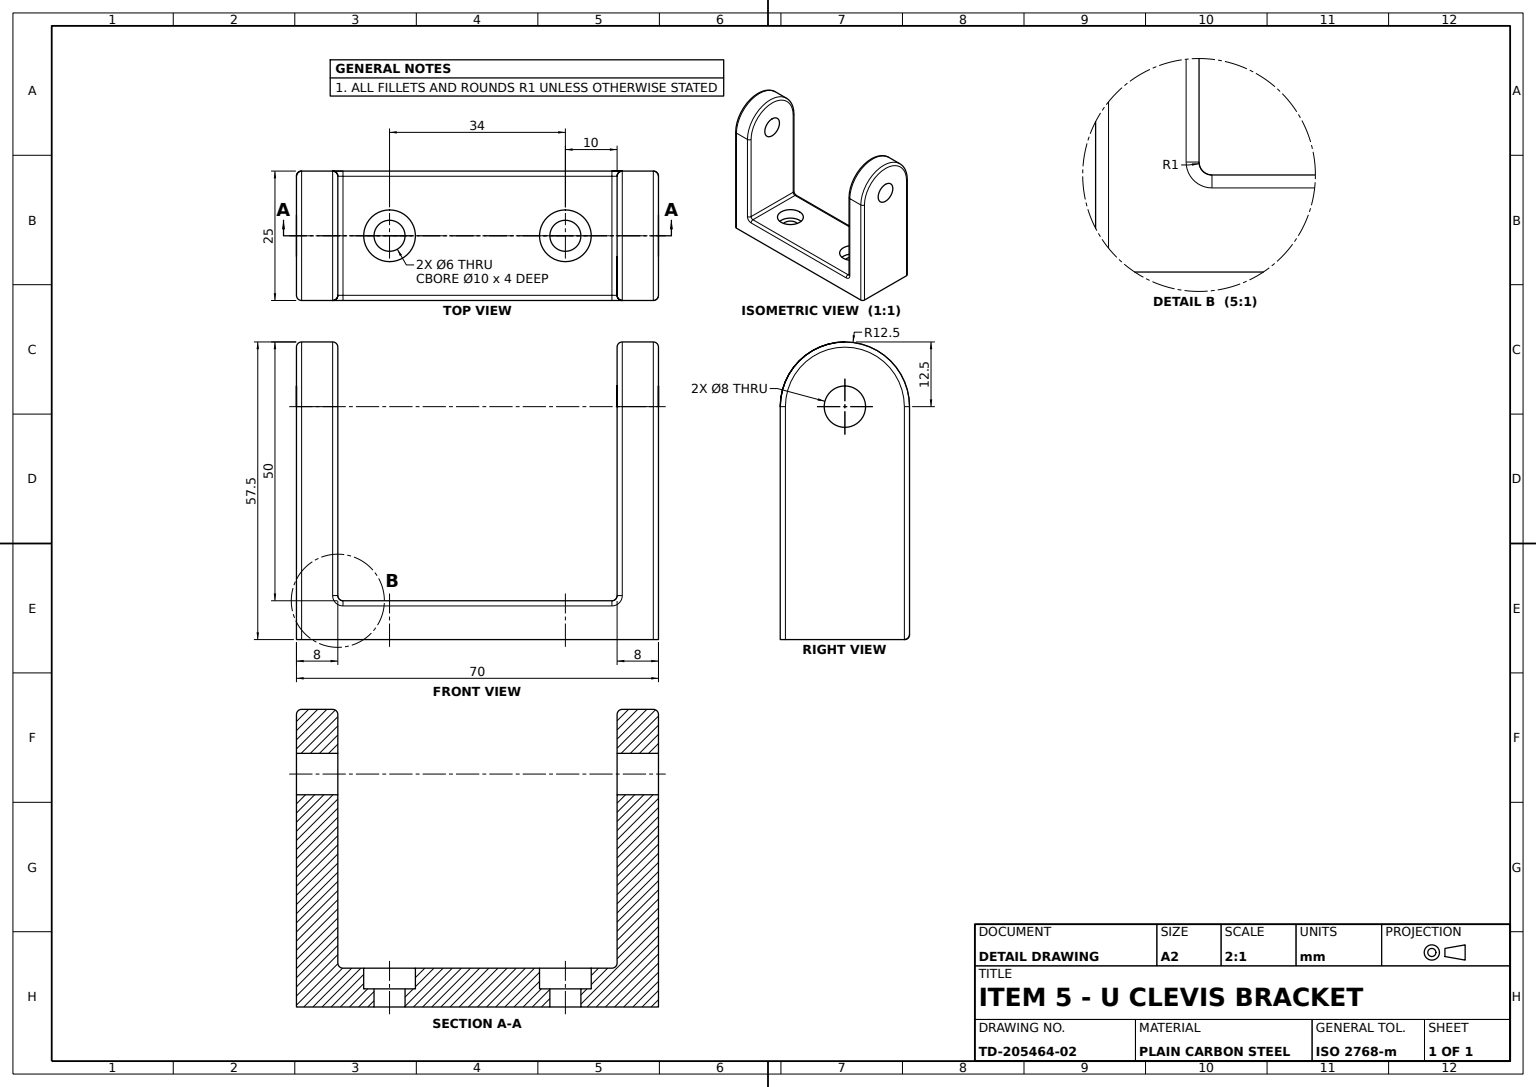
ISO-10303-21;
HEADER;
FILE_DESCRIPTION((''),'2;1');
FILE_NAME('','',(''),(''),'','','');
FILE_SCHEMA(('AUTOMOTIVE_DESIGN'));
ENDSEC;
DATA;
#1=APPLICATION_CONTEXT('');
#2=PRODUCT_CONTEXT('',#1,'mechanical');
#3=PRODUCT('','','',(#2));
#4=PRODUCT_DEFINITION_FORMATION('','',#3);
#5=PRODUCT_DEFINITION_CONTEXT('',#1,'design');
#6=PRODUCT_DEFINITION('','',#4,#5);
#7=PRODUCT_DEFINITION_SHAPE('','',#6);
#8=(LENGTH_UNIT()NAMED_UNIT(*)SI_UNIT(.MILLI.,.METRE.));
#9=(NAMED_UNIT(*)PLANE_ANGLE_UNIT()SI_UNIT($,.RADIAN.));
#10=(NAMED_UNIT(*)SI_UNIT($,.STERADIAN.)SOLID_ANGLE_UNIT());
#11=UNCERTAINTY_MEASURE_WITH_UNIT(LENGTH_MEASURE(1.E-05),#8,'distance_accuracy_value','');
#12=(GEOMETRIC_REPRESENTATION_CONTEXT(3)GLOBAL_UNCERTAINTY_ASSIGNED_CONTEXT((#11))GLOBAL_UNIT_ASSIGNED_CONTEXT((#8,#9,#10))REPRESENTATION_CONTEXT('',''));
#13=CARTESIAN_POINT('',(35.,41.,0.));
#14=VERTEX_POINT('',#13);
#15=CARTESIAN_POINT('',(35.,49.,0.));
#16=VERTEX_POINT('',#15);
#17=CARTESIAN_POINT('',(35.,45.,0.));
#18=DIRECTION('',(-1.,0.,0.));
#19=DIRECTION('',(0.,-1.,0.));
#20=AXIS2_PLACEMENT_3D('',#17,#18,#19);
#21=CIRCLE('',#20,4.);
#22=EDGE_CURVE('',#14,#16,#21,.T.);
#23=ORIENTED_EDGE('',*,*,#22,.F.);
#24=CARTESIAN_POINT('',(27.,41.,0.));
#25=VERTEX_POINT('',#24);
#26=VECTOR('',#18,1000.);
#27=LINE('',#13,#26);
#28=EDGE_CURVE('',#14,#25,#27,.T.);
#29=ORIENTED_EDGE('',*,*,#28,.T.);
#30=CARTESIAN_POINT('',(27.,49.,0.));
#31=VERTEX_POINT('',#30);
#32=CARTESIAN_POINT('',(27.,45.,0.));
#33=DIRECTION('',(1.,0.,0.));
#34=DIRECTION('',(0.,1.,0.));
#35=AXIS2_PLACEMENT_3D('',#32,#33,#34);
#36=CIRCLE('',#35,4.);
#37=EDGE_CURVE('',#31,#25,#36,.T.);
#38=ORIENTED_EDGE('',*,*,#37,.F.);
#39=LINE('',#15,#26);
#40=EDGE_CURVE('',#16,#31,#39,.T.);
#41=ORIENTED_EDGE('',*,*,#40,.F.);
#42=EDGE_LOOP('',(#23,#29,#38,#41));
#43=FACE_OUTER_BOUND('',#42,.T.);
#44=CYLINDRICAL_SURFACE('',#20,4.);
#45=ADVANCED_FACE('',(#43),#44,.F.);
#46=CARTESIAN_POINT('',(-27.,49.,0.));
#47=VERTEX_POINT('',#46);
#48=CARTESIAN_POINT('',(-35.,49.,0.));
#49=VERTEX_POINT('',#48);
#50=EDGE_CURVE('',#47,#49,#39,.T.);
#51=ORIENTED_EDGE('',*,*,#50,.F.);
#52=CARTESIAN_POINT('',(-27.,41.,0.));
#53=VERTEX_POINT('',#52);
#54=CARTESIAN_POINT('',(-27.,45.,0.));
#55=AXIS2_PLACEMENT_3D('',#54,#18,#19);
#56=CIRCLE('',#55,4.);
#57=EDGE_CURVE('',#53,#47,#56,.T.);
#58=ORIENTED_EDGE('',*,*,#57,.F.);
#59=CARTESIAN_POINT('',(-35.,41.,0.));
#60=VERTEX_POINT('',#59);
#61=EDGE_CURVE('',#53,#60,#27,.T.);
#62=ORIENTED_EDGE('',*,*,#61,.T.);
#63=CARTESIAN_POINT('',(-35.,45.,0.));
#64=AXIS2_PLACEMENT_3D('',#63,#18,#19);
#65=CIRCLE('',#64,4.);
#66=EDGE_CURVE('',#60,#49,#65,.T.);
#67=ORIENTED_EDGE('',*,*,#66,.T.);
#68=EDGE_LOOP('',(#51,#58,#62,#67));
#69=FACE_OUTER_BOUND('',#68,.T.);
#70=ADVANCED_FACE('',(#69),#44,.F.);
#71=CARTESIAN_POINT('',(-35.,0.,-11.5));
#72=VERTEX_POINT('',#71);
#73=CARTESIAN_POINT('',(35.,0.,-11.5));
#74=VERTEX_POINT('',#73);
#75=VECTOR('',#33,1000.);
#76=LINE('',#73,#75);
#77=EDGE_CURVE('',#72,#74,#76,.T.);
#78=ORIENTED_EDGE('',*,*,#77,.F.);
#79=CARTESIAN_POINT('',(-34.,1.,-12.5));
#80=VERTEX_POINT('',#79);
#81=CARTESIAN_POINT('',(-34.585786,0.414214,-12.5));
#82=CARTESIAN_POINT('',(-35.,0.,-12.085786));
#83=(BOUNDED_CURVE()B_SPLINE_CURVE(3,(#79,#81,#82,#71),.UNSPECIFIED.,.F.,.T.)B_SPLINE_CURVE_WITH_KNOTS((4,4),(1.570796327,3.141592654),.UNSPECIFIED.)CURVE()GEOMETRIC_REPRESENTATION_ITEM()RATIONAL_B_SPLINE_CURVE((1.,0.804737854,0.804737854,1.))REPRESENTATION_ITEM(''));
#84=EDGE_CURVE('',#80,#72,#83,.T.);
#85=ORIENTED_EDGE('',*,*,#84,.F.);
#86=CARTESIAN_POINT('',(34.,1.,-12.5));
#87=VERTEX_POINT('',#86);
#88=CARTESIAN_POINT('',(0.,1.,-12.5));
#89=LINE('',#88,#26);
#90=EDGE_CURVE('',#87,#80,#89,.T.);
#91=ORIENTED_EDGE('',*,*,#90,.F.);
#92=CARTESIAN_POINT('',(34.585786,0.414214,-12.5));
#93=CARTESIAN_POINT('',(35.,0.,-12.085786));
#94=(BOUNDED_CURVE()B_SPLINE_CURVE(3,(#86,#92,#93,#73),.UNSPECIFIED.,.F.,.F.)B_SPLINE_CURVE_WITH_KNOTS((4,4),(1.570796327,3.141592654),.UNSPECIFIED.)CURVE()GEOMETRIC_REPRESENTATION_ITEM()RATIONAL_B_SPLINE_CURVE((1.,0.804737854,0.804737854,1.))REPRESENTATION_ITEM(''));
#95=EDGE_CURVE('',#87,#74,#94,.T.);
#96=ORIENTED_EDGE('',*,*,#95,.T.);
#97=EDGE_LOOP('',(#78,#85,#91,#96));
#98=FACE_OUTER_BOUND('',#97,.T.);
#99=CARTESIAN_POINT('',(35.,1.,-11.5));
#100=AXIS2_PLACEMENT_3D('',#99,#33,#34);
#101=CYLINDRICAL_SURFACE('',#100,1.);
#102=ADVANCED_FACE('',(#98),#101,.T.);
#103=CARTESIAN_POINT('',(28.,8.5,-12.5));
#104=VERTEX_POINT('',#103);
#105=CARTESIAN_POINT('',(26.,6.5,-12.5));
#106=VERTEX_POINT('',#105);
#107=CARTESIAN_POINT('',(26.,8.5,-12.5));
#108=DIRECTION('',(0.,0.,-1.));
#109=AXIS2_PLACEMENT_3D('',#107,#108,#33);
#110=CIRCLE('',#109,2.);
#111=EDGE_CURVE('',#104,#106,#110,.T.);
#112=ORIENTED_EDGE('',*,*,#111,.F.);
#113=CARTESIAN_POINT('',(28.,45.,-12.5));
#114=VERTEX_POINT('',#113);
#115=CARTESIAN_POINT('',(28.,0.,-12.5));
#116=VECTOR('',#34,1000.);
#117=LINE('',#115,#116);
#118=EDGE_CURVE('',#104,#114,#117,.T.);
#119=ORIENTED_EDGE('',*,*,#118,.T.);
#120=CARTESIAN_POINT('',(34.,45.,-12.5));
#121=VERTEX_POINT('',#120);
#122=CARTESIAN_POINT('',(0.,45.,-12.5));
#123=LINE('',#122,#75);
#124=EDGE_CURVE('',#114,#121,#123,.T.);
#125=ORIENTED_EDGE('',*,*,#124,.T.);
#126=CARTESIAN_POINT('',(34.,0.,-12.5));
#127=VECTOR('',#19,1000.);
#128=LINE('',#126,#127);
#129=EDGE_CURVE('',#121,#87,#128,.T.);
#130=ORIENTED_EDGE('',*,*,#129,.T.);
#131=ORIENTED_EDGE('',*,*,#90,.T.);
#132=CARTESIAN_POINT('',(-34.,45.,-12.5));
#133=VERTEX_POINT('',#132);
#134=CARTESIAN_POINT('',(-34.,0.,-12.5));
#135=LINE('',#134,#116);
#136=EDGE_CURVE('',#80,#133,#135,.T.);
#137=ORIENTED_EDGE('',*,*,#136,.T.);
#138=CARTESIAN_POINT('',(-28.,45.,-12.5));
#139=VERTEX_POINT('',#138);
#140=EDGE_CURVE('',#133,#139,#123,.T.);
#141=ORIENTED_EDGE('',*,*,#140,.T.);
#142=CARTESIAN_POINT('',(-28.,8.5,-12.5));
#143=VERTEX_POINT('',#142);
#144=CARTESIAN_POINT('',(-28.,0.,-12.5));
#145=LINE('',#144,#127);
#146=EDGE_CURVE('',#139,#143,#145,.T.);
#147=ORIENTED_EDGE('',*,*,#146,.T.);
#148=CARTESIAN_POINT('',(-26.,6.5,-12.5));
#149=VERTEX_POINT('',#148);
#150=CARTESIAN_POINT('',(-26.,8.5,-12.5));
#151=AXIS2_PLACEMENT_3D('',#150,#108,#33);
#152=CIRCLE('',#151,2.);
#153=EDGE_CURVE('',#149,#143,#152,.T.);
#154=ORIENTED_EDGE('',*,*,#153,.F.);
#155=CARTESIAN_POINT('',(0.,6.5,-12.5));
#156=LINE('',#155,#75);
#157=EDGE_CURVE('',#149,#106,#156,.T.);
#158=ORIENTED_EDGE('',*,*,#157,.T.);
#159=EDGE_LOOP('',(#112,#119,#125,#130,#131,#137,#141,#147,#154,#158));
#160=FACE_OUTER_BOUND('',#159,.T.);
#161=CARTESIAN_POINT('',(0.,0.,-12.5));
#162=DIRECTION('',(0.,0.,1.));
#163=AXIS2_PLACEMENT_3D('',#161,#162,#33);
#164=PLANE('',#163);
#165=ADVANCED_FACE('',(#160),#164,.F.);
#166=CARTESIAN_POINT('',(17.,0.,3.));
#167=VERTEX_POINT('',#166);
#168=CARTESIAN_POINT('',(17.,3.5,3.));
#169=VERTEX_POINT('',#168);
#170=LINE('',#166,#116);
#171=EDGE_CURVE('',#167,#169,#170,.T.);
#172=ORIENTED_EDGE('',*,*,#171,.F.);
#173=CARTESIAN_POINT('',(17.,0.,-3.));
#174=VERTEX_POINT('',#173);
#175=CARTESIAN_POINT('',(17.,0.,0.));
#176=AXIS2_PLACEMENT_3D('',#175,#34,#162);
#177=CIRCLE('',#176,3.);
#178=EDGE_CURVE('',#174,#167,#177,.T.);
#179=ORIENTED_EDGE('',*,*,#178,.F.);
#180=CARTESIAN_POINT('',(17.,3.5,-3.));
#181=VERTEX_POINT('',#180);
#182=LINE('',#173,#116);
#183=EDGE_CURVE('',#174,#181,#182,.T.);
#184=ORIENTED_EDGE('',*,*,#183,.T.);
#185=CARTESIAN_POINT('',(17.,3.5,0.));
#186=AXIS2_PLACEMENT_3D('',#185,#34,#162);
#187=CIRCLE('',#186,3.);
#188=EDGE_CURVE('',#181,#169,#187,.T.);
#189=ORIENTED_EDGE('',*,*,#188,.T.);
#190=EDGE_LOOP('',(#172,#179,#184,#189));
#191=FACE_OUTER_BOUND('',#190,.T.);
#192=CYLINDRICAL_SURFACE('',#176,3.);
#193=ADVANCED_FACE('',(#191),#192,.F.);
#194=CARTESIAN_POINT('',(-34.,0.,12.5));
#195=VERTEX_POINT('',#194);
#196=CARTESIAN_POINT('',(-35.,0.,11.5));
#197=VERTEX_POINT('',#196);
#198=CARTESIAN_POINT('',(-34.,0.,11.5));
#199=AXIS2_PLACEMENT_3D('',#198,#19,#18);
#200=CIRCLE('',#199,1.);
#201=EDGE_CURVE('',#195,#197,#200,.T.);
#202=ORIENTED_EDGE('',*,*,#201,.F.);
#203=CARTESIAN_POINT('',(-34.,45.,12.5));
#204=VERTEX_POINT('',#203);
#205=LINE('',#194,#127);
#206=EDGE_CURVE('',#204,#195,#205,.T.);
#207=ORIENTED_EDGE('',*,*,#206,.F.);
#208=CARTESIAN_POINT('',(-35.,45.,11.5));
#209=VERTEX_POINT('',#208);
#210=CARTESIAN_POINT('',(-34.,45.,11.5));
#211=AXIS2_PLACEMENT_3D('',#210,#19,#108);
#212=CIRCLE('',#211,1.);
#213=EDGE_CURVE('',#204,#209,#212,.T.);
#214=ORIENTED_EDGE('',*,*,#213,.T.);
#215=LINE('',#208,#116);
#216=EDGE_CURVE('',#197,#209,#215,.T.);
#217=ORIENTED_EDGE('',*,*,#216,.F.);
#218=EDGE_LOOP('',(#202,#207,#214,#217));
#219=FACE_OUTER_BOUND('',#218,.T.);
#220=AXIS2_PLACEMENT_3D('',#198,#34,#162);
#221=CYLINDRICAL_SURFACE('',#220,1.);
#222=ADVANCED_FACE('',(#219),#221,.T.);
#223=CARTESIAN_POINT('',(34.,57.5,0.));
#224=VERTEX_POINT('',#223);
#225=CARTESIAN_POINT('',(34.,45.,0.));
#226=AXIS2_PLACEMENT_3D('',#225,#18,#162);
#227=CIRCLE('',#226,12.5);
#228=EDGE_CURVE('',#224,#121,#227,.T.);
#229=ORIENTED_EDGE('',*,*,#228,.T.);
#230=ORIENTED_EDGE('',*,*,#124,.F.);
#231=CARTESIAN_POINT('',(28.,57.5,0.));
#232=VERTEX_POINT('',#231);
#233=CARTESIAN_POINT('',(28.,45.,0.));
#234=AXIS2_PLACEMENT_3D('',#233,#33,#34);
#235=CIRCLE('',#234,12.5);
#236=EDGE_CURVE('',#114,#232,#235,.T.);
#237=ORIENTED_EDGE('',*,*,#236,.T.);
#238=CARTESIAN_POINT('',(35.,57.5,0.));
#239=LINE('',#238,#26);
#240=EDGE_CURVE('',#224,#232,#239,.T.);
#241=ORIENTED_EDGE('',*,*,#240,.F.);
#242=EDGE_LOOP('',(#229,#230,#237,#241));
#243=FACE_OUTER_BOUND('',#242,.T.);
#244=AXIS2_PLACEMENT_3D('',#17,#18,#162);
#245=CYLINDRICAL_SURFACE('',#244,12.5);
#246=ADVANCED_FACE('',(#243),#245,.T.);
#247=CARTESIAN_POINT('',(26.,7.5,11.5));
#248=VERTEX_POINT('',#247);
#249=CARTESIAN_POINT('',(26.,7.5,-11.5));
#250=VERTEX_POINT('',#249);
#251=CARTESIAN_POINT('',(26.,7.5,-12.5));
#252=VECTOR('',#108,1000.);
#253=LINE('',#251,#252);
#254=EDGE_CURVE('',#248,#250,#253,.T.);
#255=ORIENTED_EDGE('',*,*,#254,.F.);
#256=CARTESIAN_POINT('',(27.,8.5,11.5));
#257=VERTEX_POINT('',#256);
#258=CARTESIAN_POINT('',(26.,8.5,11.5));
#259=AXIS2_PLACEMENT_3D('',#258,#108,#33);
#260=CIRCLE('',#259,1.);
#261=EDGE_CURVE('',#257,#248,#260,.T.);
#262=ORIENTED_EDGE('',*,*,#261,.F.);
#263=CARTESIAN_POINT('',(27.,8.5,-11.5));
#264=VERTEX_POINT('',#263);
#265=CARTESIAN_POINT('',(27.,8.5,12.5));
#266=VECTOR('',#162,1000.);
#267=LINE('',#265,#266);
#268=EDGE_CURVE('',#264,#257,#267,.T.);
#269=ORIENTED_EDGE('',*,*,#268,.F.);
#270=CARTESIAN_POINT('',(26.,8.5,-11.5));
#271=AXIS2_PLACEMENT_3D('',#270,#108,#33);
#272=CIRCLE('',#271,1.);
#273=EDGE_CURVE('',#264,#250,#272,.T.);
#274=ORIENTED_EDGE('',*,*,#273,.T.);
#275=EDGE_LOOP('',(#255,#262,#269,#274));
#276=FACE_OUTER_BOUND('',#275,.T.);
#277=CARTESIAN_POINT('',(26.,8.5,12.5));
#278=AXIS2_PLACEMENT_3D('',#277,#162,#33);
#279=CYLINDRICAL_SURFACE('',#278,1.);
#280=ADVANCED_FACE('',(#276),#279,.F.);
#281=CARTESIAN_POINT('',(-17.,3.5,3.));
#282=VERTEX_POINT('',#281);
#283=CARTESIAN_POINT('',(-17.,3.5,-3.));
#284=VERTEX_POINT('',#283);
#285=CARTESIAN_POINT('',(-17.,3.5,0.));
#286=AXIS2_PLACEMENT_3D('',#285,#34,#162);
#287=CIRCLE('',#286,3.);
#288=EDGE_CURVE('',#282,#284,#287,.T.);
#289=ORIENTED_EDGE('',*,*,#288,.F.);
#290=EDGE_CURVE('',#284,#282,#287,.T.);
#291=ORIENTED_EDGE('',*,*,#290,.F.);
#292=EDGE_LOOP('',(#289,#291));
#293=FACE_BOUND('',#292,.T.);
#294=CARTESIAN_POINT('',(-17.,3.5,-5.));
#295=VERTEX_POINT('',#294);
#296=CARTESIAN_POINT('',(-17.,3.5,5.));
#297=VERTEX_POINT('',#296);
#298=CIRCLE('',#286,5.);
#299=EDGE_CURVE('',#295,#297,#298,.T.);
#300=ORIENTED_EDGE('',*,*,#299,.T.);
#301=EDGE_CURVE('',#297,#295,#298,.T.);
#302=ORIENTED_EDGE('',*,*,#301,.T.);
#303=EDGE_LOOP('',(#300,#302));
#304=FACE_OUTER_BOUND('',#303,.T.);
#305=PLANE('',#286);
#306=ADVANCED_FACE('',(#293,#304),#305,.T.);
#307=CARTESIAN_POINT('',(34.,0.,12.5));
#308=VERTEX_POINT('',#307);
#309=CARTESIAN_POINT('',(35.,0.,12.5));
#310=LINE('',#309,#75);
#311=EDGE_CURVE('',#195,#308,#310,.T.);
#312=ORIENTED_EDGE('',*,*,#311,.F.);
#313=ORIENTED_EDGE('',*,*,#201,.T.);
#314=CARTESIAN_POINT('',(-35.,0.,12.5));
#315=LINE('',#314,#252);
#316=EDGE_CURVE('',#197,#72,#315,.T.);
#317=ORIENTED_EDGE('',*,*,#316,.T.);
#318=ORIENTED_EDGE('',*,*,#77,.T.);
#319=CARTESIAN_POINT('',(35.,0.,11.5));
#320=VERTEX_POINT('',#319);
#321=LINE('',#309,#252);
#322=EDGE_CURVE('',#320,#74,#321,.T.);
#323=ORIENTED_EDGE('',*,*,#322,.F.);
#324=CARTESIAN_POINT('',(34.,0.,11.5));
#325=AXIS2_PLACEMENT_3D('',#324,#19,#18);
#326=CIRCLE('',#325,1.);
#327=EDGE_CURVE('',#320,#308,#326,.T.);
#328=ORIENTED_EDGE('',*,*,#327,.T.);
#329=EDGE_LOOP('',(#312,#313,#317,#318,#323,#328));
#330=FACE_OUTER_BOUND('',#329,.T.);
#331=ORIENTED_EDGE('',*,*,#178,.T.);
#332=EDGE_CURVE('',#167,#174,#177,.T.);
#333=ORIENTED_EDGE('',*,*,#332,.T.);
#334=EDGE_LOOP('',(#331,#333));
#335=FACE_BOUND('',#334,.T.);
#336=CARTESIAN_POINT('',(-17.,0.,3.));
#337=VERTEX_POINT('',#336);
#338=CARTESIAN_POINT('',(-17.,0.,-3.));
#339=VERTEX_POINT('',#338);
#340=CARTESIAN_POINT('',(-17.,0.,0.));
#341=AXIS2_PLACEMENT_3D('',#340,#34,#162);
#342=CIRCLE('',#341,3.);
#343=EDGE_CURVE('',#337,#339,#342,.T.);
#344=ORIENTED_EDGE('',*,*,#343,.T.);
#345=EDGE_CURVE('',#339,#337,#342,.T.);
#346=ORIENTED_EDGE('',*,*,#345,.T.);
#347=EDGE_LOOP('',(#344,#346));
#348=FACE_BOUND('',#347,.T.);
#349=AXIS2_PLACEMENT_3D('',#309,#34,#18);
#350=PLANE('',#349);
#351=ADVANCED_FACE('',(#330,#335,#348),#350,.F.);
#352=CARTESIAN_POINT('',(-35.,56.5,0.));
#353=VERTEX_POINT('',#352);
#354=AXIS2_PLACEMENT_3D('',#63,#18,#108);
#355=CIRCLE('',#354,11.5);
#356=EDGE_CURVE('',#209,#353,#355,.T.);
#357=ORIENTED_EDGE('',*,*,#356,.F.);
#358=ORIENTED_EDGE('',*,*,#213,.F.);
#359=CARTESIAN_POINT('',(-34.,57.5,0.));
#360=VERTEX_POINT('',#359);
#361=CARTESIAN_POINT('',(-34.,45.,0.));
#362=AXIS2_PLACEMENT_3D('',#361,#33,#108);
#363=CIRCLE('',#362,12.5);
#364=EDGE_CURVE('',#360,#204,#363,.T.);
#365=ORIENTED_EDGE('',*,*,#364,.F.);
#366=CARTESIAN_POINT('',(-34.,56.5,0.));
#367=AXIS2_PLACEMENT_3D('',#366,#162,#33);
#368=CIRCLE('',#367,1.);
#369=EDGE_CURVE('',#360,#353,#368,.T.);
#370=ORIENTED_EDGE('',*,*,#369,.T.);
#371=EDGE_LOOP('',(#357,#358,#365,#370));
#372=FACE_OUTER_BOUND('',#371,.T.);
#373=TOROIDAL_SURFACE('',#362,11.5,1.);
#374=ADVANCED_FACE('',(#372),#373,.T.);
#375=CARTESIAN_POINT('',(27.,45.,-11.5));
#376=VERTEX_POINT('',#375);
#377=CARTESIAN_POINT('',(27.,57.5,-11.5));
#378=LINE('',#377,#127);
#379=EDGE_CURVE('',#376,#264,#378,.T.);
#380=ORIENTED_EDGE('',*,*,#379,.F.);
#381=CARTESIAN_POINT('',(28.,45.,-11.5));
#382=AXIS2_PLACEMENT_3D('',#381,#34,#162);
#383=CIRCLE('',#382,1.);
#384=EDGE_CURVE('',#114,#376,#383,.T.);
#385=ORIENTED_EDGE('',*,*,#384,.F.);
#386=ORIENTED_EDGE('',*,*,#118,.F.);
#387=CARTESIAN_POINT('',(28.,8.5,-11.5));
#388=AXIS2_PLACEMENT_3D('',#387,#19,#108);
#389=CIRCLE('',#388,1.);
#390=EDGE_CURVE('',#264,#104,#389,.T.);
#391=ORIENTED_EDGE('',*,*,#390,.F.);
#392=EDGE_LOOP('',(#380,#385,#386,#391));
#393=FACE_OUTER_BOUND('',#392,.T.);
#394=CARTESIAN_POINT('',(28.,57.5,-11.5));
#395=AXIS2_PLACEMENT_3D('',#394,#19,#33);
#396=CYLINDRICAL_SURFACE('',#395,1.);
#397=ADVANCED_FACE('',(#393),#396,.T.);
#398=CARTESIAN_POINT('',(-26.,7.5,-11.5));
#399=VERTEX_POINT('',#398);
#400=CARTESIAN_POINT('',(-27.,7.5,-11.5));
#401=LINE('',#400,#26);
#402=EDGE_CURVE('',#250,#399,#401,.T.);
#403=ORIENTED_EDGE('',*,*,#402,.F.);
#404=CARTESIAN_POINT('',(26.,6.5,-11.5));
#405=AXIS2_PLACEMENT_3D('',#404,#18,#108);
#406=CIRCLE('',#405,1.);
#407=EDGE_CURVE('',#250,#106,#406,.T.);
#408=ORIENTED_EDGE('',*,*,#407,.T.);
#409=ORIENTED_EDGE('',*,*,#157,.F.);
#410=CARTESIAN_POINT('',(-26.,6.5,-11.5));
#411=AXIS2_PLACEMENT_3D('',#410,#18,#162);
#412=CIRCLE('',#411,1.);
#413=EDGE_CURVE('',#399,#149,#412,.T.);
#414=ORIENTED_EDGE('',*,*,#413,.F.);
#415=EDGE_LOOP('',(#403,#408,#409,#414));
#416=FACE_OUTER_BOUND('',#415,.T.);
#417=CARTESIAN_POINT('',(-27.,6.5,-11.5));
#418=AXIS2_PLACEMENT_3D('',#417,#18,#162);
#419=CYLINDRICAL_SURFACE('',#418,1.);
#420=ADVANCED_FACE('',(#416),#419,.T.);
#421=ORIENTED_EDGE('',*,*,#22,.T.);
#422=EDGE_CURVE('',#16,#14,#21,.T.);
#423=ORIENTED_EDGE('',*,*,#422,.T.);
#424=EDGE_LOOP('',(#421,#423));
#425=FACE_BOUND('',#424,.T.);
#426=CARTESIAN_POINT('',(35.,45.,-11.5));
#427=VERTEX_POINT('',#426);
#428=CARTESIAN_POINT('',(35.,56.5,0.));
#429=VERTEX_POINT('',#428);
#430=AXIS2_PLACEMENT_3D('',#17,#33,#162);
#431=CIRCLE('',#430,11.5);
#432=EDGE_CURVE('',#427,#429,#431,.T.);
#433=ORIENTED_EDGE('',*,*,#432,.T.);
#434=CARTESIAN_POINT('',(35.,45.,11.5));
#435=VERTEX_POINT('',#434);
#436=EDGE_CURVE('',#429,#435,#431,.T.);
#437=ORIENTED_EDGE('',*,*,#436,.T.);
#438=LINE('',#319,#127);
#439=EDGE_CURVE('',#435,#320,#438,.T.);
#440=ORIENTED_EDGE('',*,*,#439,.T.);
#441=ORIENTED_EDGE('',*,*,#322,.T.);
#442=LINE('',#73,#116);
#443=EDGE_CURVE('',#74,#427,#442,.T.);
#444=ORIENTED_EDGE('',*,*,#443,.T.);
#445=EDGE_LOOP('',(#433,#437,#440,#441,#444));
#446=FACE_OUTER_BOUND('',#445,.T.);
#447=AXIS2_PLACEMENT_3D('',#309,#18,#162);
#448=PLANE('',#447);
#449=ADVANCED_FACE('',(#425,#446),#448,.F.);
#450=ORIENTED_EDGE('',*,*,#443,.F.);
#451=ORIENTED_EDGE('',*,*,#95,.F.);
#452=ORIENTED_EDGE('',*,*,#129,.F.);
#453=CARTESIAN_POINT('',(34.,45.,-11.5));
#454=AXIS2_PLACEMENT_3D('',#453,#19,#108);
#455=CIRCLE('',#454,1.);
#456=EDGE_CURVE('',#121,#427,#455,.T.);
#457=ORIENTED_EDGE('',*,*,#456,.T.);
#458=EDGE_LOOP('',(#450,#451,#452,#457));
#459=FACE_OUTER_BOUND('',#458,.T.);
#460=CARTESIAN_POINT('',(34.,0.,-11.5));
#461=AXIS2_PLACEMENT_3D('',#460,#34,#162);
#462=CYLINDRICAL_SURFACE('',#461,1.);
#463=ADVANCED_FACE('',(#459),#462,.T.);
#464=CARTESIAN_POINT('',(-17.,7.5,-5.));
#465=VERTEX_POINT('',#464);
#466=CARTESIAN_POINT('',(-17.,7.5,5.));
#467=VERTEX_POINT('',#466);
#468=CARTESIAN_POINT('',(-17.,7.5,0.));
#469=AXIS2_PLACEMENT_3D('',#468,#34,#162);
#470=CIRCLE('',#469,5.);
#471=EDGE_CURVE('',#465,#467,#470,.T.);
#472=ORIENTED_EDGE('',*,*,#471,.T.);
#473=LINE('',#296,#116);
#474=EDGE_CURVE('',#297,#467,#473,.T.);
#475=ORIENTED_EDGE('',*,*,#474,.F.);
#476=ORIENTED_EDGE('',*,*,#299,.F.);
#477=LINE('',#294,#116);
#478=EDGE_CURVE('',#295,#465,#477,.T.);
#479=ORIENTED_EDGE('',*,*,#478,.T.);
#480=EDGE_LOOP('',(#472,#475,#476,#479));
#481=FACE_OUTER_BOUND('',#480,.T.);
#482=CYLINDRICAL_SURFACE('',#286,5.);
#483=ADVANCED_FACE('',(#481),#482,.F.);
#484=ORIENTED_EDGE('',*,*,#57,.T.);
#485=EDGE_CURVE('',#47,#53,#56,.T.);
#486=ORIENTED_EDGE('',*,*,#485,.T.);
#487=EDGE_LOOP('',(#484,#486));
#488=FACE_BOUND('',#487,.T.);
#489=CARTESIAN_POINT('',(-27.,8.5,11.5));
#490=VERTEX_POINT('',#489);
#491=CARTESIAN_POINT('',(-27.,8.5,-11.5));
#492=VERTEX_POINT('',#491);
#493=CARTESIAN_POINT('',(-27.,8.5,-12.5));
#494=LINE('',#493,#252);
#495=EDGE_CURVE('',#490,#492,#494,.T.);
#496=ORIENTED_EDGE('',*,*,#495,.T.);
#497=CARTESIAN_POINT('',(-27.,45.,-11.5));
#498=VERTEX_POINT('',#497);
#499=CARTESIAN_POINT('',(-27.,57.5,-11.5));
#500=LINE('',#499,#116);
#501=EDGE_CURVE('',#492,#498,#500,.T.);
#502=ORIENTED_EDGE('',*,*,#501,.T.);
#503=CARTESIAN_POINT('',(-27.,56.5,0.));
#504=VERTEX_POINT('',#503);
#505=AXIS2_PLACEMENT_3D('',#54,#33,#19);
#506=CIRCLE('',#505,11.5);
#507=EDGE_CURVE('',#498,#504,#506,.T.);
#508=ORIENTED_EDGE('',*,*,#507,.T.);
#509=CARTESIAN_POINT('',(-27.,45.,11.5));
#510=VERTEX_POINT('',#509);
#511=EDGE_CURVE('',#504,#510,#506,.T.);
#512=ORIENTED_EDGE('',*,*,#511,.T.);
#513=CARTESIAN_POINT('',(-27.,7.5,11.5));
#514=LINE('',#513,#127);
#515=EDGE_CURVE('',#510,#490,#514,.T.);
#516=ORIENTED_EDGE('',*,*,#515,.T.);
#517=EDGE_LOOP('',(#496,#502,#508,#512,#516));
#518=FACE_OUTER_BOUND('',#517,.T.);
#519=CARTESIAN_POINT('',(-27.,57.5,12.5));
#520=AXIS2_PLACEMENT_3D('',#519,#18,#19);
#521=PLANE('',#520);
#522=ADVANCED_FACE('',(#488,#518),#521,.F.);
#523=CARTESIAN_POINT('',(27.,56.5,0.));
#524=VERTEX_POINT('',#523);
#525=CARTESIAN_POINT('',(28.,56.5,0.));
#526=AXIS2_PLACEMENT_3D('',#525,#162,#33);
#527=CIRCLE('',#526,1.);
#528=EDGE_CURVE('',#232,#524,#527,.T.);
#529=ORIENTED_EDGE('',*,*,#528,.T.);
#530=CARTESIAN_POINT('',(27.,45.,11.5));
#531=VERTEX_POINT('',#530);
#532=AXIS2_PLACEMENT_3D('',#32,#18,#34);
#533=CIRCLE('',#532,11.5);
#534=EDGE_CURVE('',#531,#524,#533,.T.);
#535=ORIENTED_EDGE('',*,*,#534,.F.);
#536=CARTESIAN_POINT('',(28.,45.,12.5));
#537=VERTEX_POINT('',#536);
#538=CARTESIAN_POINT('',(28.,45.,11.5));
#539=AXIS2_PLACEMENT_3D('',#538,#19,#108);
#540=CIRCLE('',#539,1.);
#541=EDGE_CURVE('',#537,#531,#540,.T.);
#542=ORIENTED_EDGE('',*,*,#541,.F.);
#543=EDGE_CURVE('',#232,#537,#235,.T.);
#544=ORIENTED_EDGE('',*,*,#543,.F.);
#545=EDGE_LOOP('',(#529,#535,#542,#544));
#546=FACE_OUTER_BOUND('',#545,.T.);
#547=TOROIDAL_SURFACE('',#234,11.5,1.);
#548=ADVANCED_FACE('',(#546),#547,.T.);
#549=CARTESIAN_POINT('',(17.,3.5,5.));
#550=VERTEX_POINT('',#549);
#551=CARTESIAN_POINT('',(17.,7.5,5.));
#552=VERTEX_POINT('',#551);
#553=LINE('',#549,#116);
#554=EDGE_CURVE('',#550,#552,#553,.T.);
#555=ORIENTED_EDGE('',*,*,#554,.T.);
#556=CARTESIAN_POINT('',(17.,7.5,-5.));
#557=VERTEX_POINT('',#556);
#558=CARTESIAN_POINT('',(17.,7.5,0.));
#559=AXIS2_PLACEMENT_3D('',#558,#34,#162);
#560=CIRCLE('',#559,5.);
#561=EDGE_CURVE('',#552,#557,#560,.T.);
#562=ORIENTED_EDGE('',*,*,#561,.T.);
#563=CARTESIAN_POINT('',(17.,3.5,-5.));
#564=VERTEX_POINT('',#563);
#565=LINE('',#563,#116);
#566=EDGE_CURVE('',#564,#557,#565,.T.);
#567=ORIENTED_EDGE('',*,*,#566,.F.);
#568=CIRCLE('',#186,5.);
#569=EDGE_CURVE('',#550,#564,#568,.T.);
#570=ORIENTED_EDGE('',*,*,#569,.F.);
#571=EDGE_LOOP('',(#555,#562,#567,#570));
#572=FACE_OUTER_BOUND('',#571,.T.);
#573=CYLINDRICAL_SURFACE('',#186,5.);
#574=ADVANCED_FACE('',(#572),#573,.F.);
#575=ORIENTED_EDGE('',*,*,#379,.T.);
#576=ORIENTED_EDGE('',*,*,#268,.T.);
#577=LINE('',#530,#116);
#578=EDGE_CURVE('',#257,#531,#577,.T.);
#579=ORIENTED_EDGE('',*,*,#578,.T.);
#580=ORIENTED_EDGE('',*,*,#534,.T.);
#581=EDGE_CURVE('',#524,#376,#533,.T.);
#582=ORIENTED_EDGE('',*,*,#581,.T.);
#583=EDGE_LOOP('',(#575,#576,#579,#580,#582));
#584=FACE_OUTER_BOUND('',#583,.T.);
#585=EDGE_CURVE('',#25,#31,#36,.T.);
#586=ORIENTED_EDGE('',*,*,#585,.T.);
#587=ORIENTED_EDGE('',*,*,#37,.T.);
#588=EDGE_LOOP('',(#586,#587));
#589=FACE_BOUND('',#588,.T.);
#590=CARTESIAN_POINT('',(27.,57.5,12.5));
#591=AXIS2_PLACEMENT_3D('',#590,#33,#34);
#592=PLANE('',#591);
#593=ADVANCED_FACE('',(#584,#589),#592,.F.);
#594=CARTESIAN_POINT('',(-28.,8.5,12.5));
#595=VERTEX_POINT('',#594);
#596=CARTESIAN_POINT('',(-26.,6.5,12.5));
#597=VERTEX_POINT('',#596);
#598=CARTESIAN_POINT('',(-26.,8.5,12.5));
#599=AXIS2_PLACEMENT_3D('',#598,#162,#33);
#600=CIRCLE('',#599,2.);
#601=EDGE_CURVE('',#595,#597,#600,.T.);
#602=ORIENTED_EDGE('',*,*,#601,.T.);
#603=CARTESIAN_POINT('',(-26.,7.5,11.5));
#604=VERTEX_POINT('',#603);
#605=CARTESIAN_POINT('',(-26.,6.5,11.5));
#606=AXIS2_PLACEMENT_3D('',#605,#18,#162);
#607=CIRCLE('',#606,1.);
#608=EDGE_CURVE('',#597,#604,#607,.T.);
#609=ORIENTED_EDGE('',*,*,#608,.T.);
#610=CARTESIAN_POINT('',(-26.,8.5,11.5));
#611=AXIS2_PLACEMENT_3D('',#610,#108,#33);
#612=CIRCLE('',#611,1.);
#613=EDGE_CURVE('',#604,#490,#612,.T.);
#614=ORIENTED_EDGE('',*,*,#613,.T.);
#615=CARTESIAN_POINT('',(-28.,8.5,11.5));
#616=AXIS2_PLACEMENT_3D('',#615,#34,#108);
#617=CIRCLE('',#616,1.);
#618=EDGE_CURVE('',#595,#490,#617,.T.);
#619=ORIENTED_EDGE('',*,*,#618,.F.);
#620=EDGE_LOOP('',(#602,#609,#614,#619));
#621=FACE_OUTER_BOUND('',#620,.T.);
#622=AXIS2_PLACEMENT_3D('',#610,#162,#33);
#623=TOROIDAL_SURFACE('',#622,2.,1.);
#624=ADVANCED_FACE('',(#621),#623,.T.);
#625=ORIENTED_EDGE('',*,*,#290,.T.);
#626=LINE('',#336,#116);
#627=EDGE_CURVE('',#337,#282,#626,.T.);
#628=ORIENTED_EDGE('',*,*,#627,.F.);
#629=ORIENTED_EDGE('',*,*,#345,.F.);
#630=LINE('',#338,#116);
#631=EDGE_CURVE('',#339,#284,#630,.T.);
#632=ORIENTED_EDGE('',*,*,#631,.T.);
#633=EDGE_LOOP('',(#625,#628,#629,#632));
#634=FACE_OUTER_BOUND('',#633,.T.);
#635=CYLINDRICAL_SURFACE('',#341,3.);
#636=ADVANCED_FACE('',(#634),#635,.F.);
#637=ORIENTED_EDGE('',*,*,#439,.F.);
#638=CARTESIAN_POINT('',(34.,45.,12.5));
#639=VERTEX_POINT('',#638);
#640=CARTESIAN_POINT('',(34.,45.,11.5));
#641=AXIS2_PLACEMENT_3D('',#640,#34,#162);
#642=CIRCLE('',#641,1.);
#643=EDGE_CURVE('',#639,#435,#642,.T.);
#644=ORIENTED_EDGE('',*,*,#643,.F.);
#645=LINE('',#638,#116);
#646=EDGE_CURVE('',#308,#639,#645,.T.);
#647=ORIENTED_EDGE('',*,*,#646,.F.);
#648=ORIENTED_EDGE('',*,*,#327,.F.);
#649=EDGE_LOOP('',(#637,#644,#647,#648));
#650=FACE_OUTER_BOUND('',#649,.T.);
#651=AXIS2_PLACEMENT_3D('',#324,#19,#108);
#652=CYLINDRICAL_SURFACE('',#651,1.);
#653=ADVANCED_FACE('',(#650),#652,.T.);
#654=EDGE_CURVE('',#133,#360,#363,.T.);
#655=ORIENTED_EDGE('',*,*,#654,.T.);
#656=CARTESIAN_POINT('',(-28.,57.5,0.));
#657=VERTEX_POINT('',#656);
#658=CARTESIAN_POINT('',(-27.,57.5,0.));
#659=LINE('',#658,#75);
#660=EDGE_CURVE('',#360,#657,#659,.T.);
#661=ORIENTED_EDGE('',*,*,#660,.T.);
#662=CARTESIAN_POINT('',(-28.,45.,0.));
#663=AXIS2_PLACEMENT_3D('',#662,#18,#19);
#664=CIRCLE('',#663,12.5);
#665=EDGE_CURVE('',#657,#139,#664,.T.);
#666=ORIENTED_EDGE('',*,*,#665,.T.);
#667=ORIENTED_EDGE('',*,*,#140,.F.);
#668=EDGE_LOOP('',(#655,#661,#666,#667));
#669=FACE_OUTER_BOUND('',#668,.T.);
#670=AXIS2_PLACEMENT_3D('',#63,#18,#162);
#671=CYLINDRICAL_SURFACE('',#670,12.5);
#672=ADVANCED_FACE('',(#669),#671,.T.);
#673=ORIENTED_EDGE('',*,*,#288,.T.);
#674=ORIENTED_EDGE('',*,*,#631,.F.);
#675=ORIENTED_EDGE('',*,*,#343,.F.);
#676=ORIENTED_EDGE('',*,*,#627,.T.);
#677=EDGE_LOOP('',(#673,#674,#675,#676));
#678=FACE_OUTER_BOUND('',#677,.T.);
#679=ADVANCED_FACE('',(#678),#635,.F.);
#680=ORIENTED_EDGE('',*,*,#422,.F.);
#681=ORIENTED_EDGE('',*,*,#40,.T.);
#682=ORIENTED_EDGE('',*,*,#585,.F.);
#683=ORIENTED_EDGE('',*,*,#28,.F.);
#684=EDGE_LOOP('',(#680,#681,#682,#683));
#685=FACE_OUTER_BOUND('',#684,.T.);
#686=ADVANCED_FACE('',(#685),#44,.F.);
#687=ORIENTED_EDGE('',*,*,#171,.T.);
#688=EDGE_CURVE('',#169,#181,#187,.T.);
#689=ORIENTED_EDGE('',*,*,#688,.T.);
#690=ORIENTED_EDGE('',*,*,#183,.F.);
#691=ORIENTED_EDGE('',*,*,#332,.F.);
#692=EDGE_LOOP('',(#687,#689,#690,#691));
#693=FACE_OUTER_BOUND('',#692,.T.);
#694=ADVANCED_FACE('',(#693),#192,.F.);
#695=CARTESIAN_POINT('',(28.,8.5,12.5));
#696=VERTEX_POINT('',#695);
#697=CARTESIAN_POINT('',(28.,7.5,12.5));
#698=LINE('',#697,#127);
#699=EDGE_CURVE('',#537,#696,#698,.T.);
#700=ORIENTED_EDGE('',*,*,#699,.F.);
#701=ORIENTED_EDGE('',*,*,#541,.T.);
#702=ORIENTED_EDGE('',*,*,#578,.F.);
#703=CARTESIAN_POINT('',(28.,8.5,11.5));
#704=AXIS2_PLACEMENT_3D('',#703,#19,#108);
#705=CIRCLE('',#704,1.);
#706=EDGE_CURVE('',#696,#257,#705,.T.);
#707=ORIENTED_EDGE('',*,*,#706,.F.);
#708=EDGE_LOOP('',(#700,#701,#702,#707));
#709=FACE_OUTER_BOUND('',#708,.T.);
#710=CARTESIAN_POINT('',(28.,0.,11.5));
#711=AXIS2_PLACEMENT_3D('',#710,#34,#18);
#712=CYLINDRICAL_SURFACE('',#711,1.);
#713=ADVANCED_FACE('',(#709),#712,.T.);
#714=ORIENTED_EDGE('',*,*,#474,.T.);
#715=EDGE_CURVE('',#467,#465,#470,.T.);
#716=ORIENTED_EDGE('',*,*,#715,.T.);
#717=ORIENTED_EDGE('',*,*,#478,.F.);
#718=ORIENTED_EDGE('',*,*,#301,.F.);
#719=EDGE_LOOP('',(#714,#716,#717,#718));
#720=FACE_OUTER_BOUND('',#719,.T.);
#721=ADVANCED_FACE('',(#720),#482,.F.);
#722=EDGE_CURVE('',#564,#550,#568,.T.);
#723=ORIENTED_EDGE('',*,*,#722,.T.);
#724=ORIENTED_EDGE('',*,*,#569,.T.);
#725=EDGE_LOOP('',(#723,#724));
#726=FACE_OUTER_BOUND('',#725,.T.);
#727=ORIENTED_EDGE('',*,*,#688,.F.);
#728=ORIENTED_EDGE('',*,*,#188,.F.);
#729=EDGE_LOOP('',(#727,#728));
#730=FACE_BOUND('',#729,.T.);
#731=PLANE('',#186);
#732=ADVANCED_FACE('',(#726,#730),#731,.T.);
#733=ORIENTED_EDGE('',*,*,#50,.T.);
#734=EDGE_CURVE('',#49,#60,#65,.T.);
#735=ORIENTED_EDGE('',*,*,#734,.T.);
#736=ORIENTED_EDGE('',*,*,#61,.F.);
#737=ORIENTED_EDGE('',*,*,#485,.F.);
#738=EDGE_LOOP('',(#733,#735,#736,#737));
#739=FACE_OUTER_BOUND('',#738,.T.);
#740=ADVANCED_FACE('',(#739),#44,.F.);
#741=ORIENTED_EDGE('',*,*,#153,.T.);
#742=CARTESIAN_POINT('',(-28.,8.5,-11.5));
#743=AXIS2_PLACEMENT_3D('',#742,#34,#108);
#744=CIRCLE('',#743,1.);
#745=EDGE_CURVE('',#492,#143,#744,.T.);
#746=ORIENTED_EDGE('',*,*,#745,.F.);
#747=CARTESIAN_POINT('',(-26.,8.5,-11.5));
#748=AXIS2_PLACEMENT_3D('',#747,#108,#33);
#749=CIRCLE('',#748,1.);
#750=EDGE_CURVE('',#399,#492,#749,.T.);
#751=ORIENTED_EDGE('',*,*,#750,.F.);
#752=ORIENTED_EDGE('',*,*,#413,.T.);
#753=EDGE_LOOP('',(#741,#746,#751,#752));
#754=FACE_OUTER_BOUND('',#753,.T.);
#755=AXIS2_PLACEMENT_3D('',#747,#162,#33);
#756=TOROIDAL_SURFACE('',#755,2.,1.);
#757=ADVANCED_FACE('',(#754),#756,.T.);
#758=ORIENTED_EDGE('',*,*,#643,.T.);
#759=ORIENTED_EDGE('',*,*,#436,.F.);
#760=CARTESIAN_POINT('',(34.,56.5,0.));
#761=AXIS2_PLACEMENT_3D('',#760,#108,#18);
#762=CIRCLE('',#761,1.);
#763=EDGE_CURVE('',#224,#429,#762,.T.);
#764=ORIENTED_EDGE('',*,*,#763,.F.);
#765=EDGE_CURVE('',#639,#224,#227,.T.);
#766=ORIENTED_EDGE('',*,*,#765,.F.);
#767=EDGE_LOOP('',(#758,#759,#764,#766));
#768=FACE_OUTER_BOUND('',#767,.T.);
#769=TOROIDAL_SURFACE('',#226,11.5,1.);
#770=ADVANCED_FACE('',(#768),#769,.T.);
#771=CARTESIAN_POINT('',(26.,6.5,12.5));
#772=VERTEX_POINT('',#771);
#773=CIRCLE('',#278,2.);
#774=EDGE_CURVE('',#772,#696,#773,.T.);
#775=ORIENTED_EDGE('',*,*,#774,.T.);
#776=ORIENTED_EDGE('',*,*,#706,.T.);
#777=ORIENTED_EDGE('',*,*,#261,.T.);
#778=CARTESIAN_POINT('',(26.,6.5,11.5));
#779=AXIS2_PLACEMENT_3D('',#778,#18,#108);
#780=CIRCLE('',#779,1.);
#781=EDGE_CURVE('',#772,#248,#780,.T.);
#782=ORIENTED_EDGE('',*,*,#781,.F.);
#783=EDGE_LOOP('',(#775,#776,#777,#782));
#784=FACE_OUTER_BOUND('',#783,.T.);
#785=AXIS2_PLACEMENT_3D('',#258,#162,#33);
#786=TOROIDAL_SURFACE('',#785,2.,1.);
#787=ADVANCED_FACE('',(#784),#786,.T.);
#788=ORIENTED_EDGE('',*,*,#734,.F.);
#789=ORIENTED_EDGE('',*,*,#66,.F.);
#790=EDGE_LOOP('',(#788,#789));
#791=FACE_BOUND('',#790,.T.);
#792=ORIENTED_EDGE('',*,*,#316,.F.);
#793=ORIENTED_EDGE('',*,*,#216,.T.);
#794=ORIENTED_EDGE('',*,*,#356,.T.);
#795=CARTESIAN_POINT('',(-35.,45.,-11.5));
#796=VERTEX_POINT('',#795);
#797=EDGE_CURVE('',#353,#796,#355,.T.);
#798=ORIENTED_EDGE('',*,*,#797,.T.);
#799=LINE('',#71,#127);
#800=EDGE_CURVE('',#796,#72,#799,.T.);
#801=ORIENTED_EDGE('',*,*,#800,.T.);
#802=EDGE_LOOP('',(#792,#793,#794,#798,#801));
#803=FACE_OUTER_BOUND('',#802,.T.);
#804=AXIS2_PLACEMENT_3D('',#314,#33,#108);
#805=PLANE('',#804);
#806=ADVANCED_FACE('',(#791,#803),#805,.F.);
#807=CARTESIAN_POINT('',(-28.,45.,12.5));
#808=VERTEX_POINT('',#807);
#809=LINE('',#807,#116);
#810=EDGE_CURVE('',#595,#808,#809,.T.);
#811=ORIENTED_EDGE('',*,*,#810,.F.);
#812=ORIENTED_EDGE('',*,*,#618,.T.);
#813=ORIENTED_EDGE('',*,*,#515,.F.);
#814=CARTESIAN_POINT('',(-28.,45.,11.5));
#815=AXIS2_PLACEMENT_3D('',#814,#19,#108);
#816=CIRCLE('',#815,1.);
#817=EDGE_CURVE('',#510,#808,#816,.T.);
#818=ORIENTED_EDGE('',*,*,#817,.T.);
#819=EDGE_LOOP('',(#811,#812,#813,#818));
#820=FACE_OUTER_BOUND('',#819,.T.);
#821=CARTESIAN_POINT('',(-28.,0.,11.5));
#822=AXIS2_PLACEMENT_3D('',#821,#19,#33);
#823=CYLINDRICAL_SURFACE('',#822,1.);
#824=ADVANCED_FACE('',(#820),#823,.T.);
#825=CARTESIAN_POINT('',(-35.,45.,12.5));
#826=LINE('',#825,#26);
#827=EDGE_CURVE('',#808,#204,#826,.T.);
#828=ORIENTED_EDGE('',*,*,#827,.F.);
#829=EDGE_CURVE('',#808,#657,#664,.T.);
#830=ORIENTED_EDGE('',*,*,#829,.T.);
#831=ORIENTED_EDGE('',*,*,#660,.F.);
#832=ORIENTED_EDGE('',*,*,#364,.T.);
#833=EDGE_LOOP('',(#828,#830,#831,#832));
#834=FACE_OUTER_BOUND('',#833,.T.);
#835=CARTESIAN_POINT('',(0.,45.,0.));
#836=AXIS2_PLACEMENT_3D('',#835,#33,#108);
#837=CYLINDRICAL_SURFACE('',#836,12.5);
#838=ADVANCED_FACE('',(#834),#837,.T.);
#839=ORIENTED_EDGE('',*,*,#781,.T.);
#840=CARTESIAN_POINT('',(27.,7.5,11.5));
#841=LINE('',#840,#75);
#842=EDGE_CURVE('',#604,#248,#841,.T.);
#843=ORIENTED_EDGE('',*,*,#842,.F.);
#844=ORIENTED_EDGE('',*,*,#608,.F.);
#845=CARTESIAN_POINT('',(-27.,6.5,12.5));
#846=LINE('',#845,#26);
#847=EDGE_CURVE('',#772,#597,#846,.T.);
#848=ORIENTED_EDGE('',*,*,#847,.F.);
#849=EDGE_LOOP('',(#839,#843,#844,#848));
#850=FACE_OUTER_BOUND('',#849,.T.);
#851=CARTESIAN_POINT('',(0.,6.5,11.5));
#852=AXIS2_PLACEMENT_3D('',#851,#33,#108);
#853=CYLINDRICAL_SURFACE('',#852,1.);
#854=ADVANCED_FACE('',(#850),#853,.T.);
#855=ORIENTED_EDGE('',*,*,#384,.T.);
#856=ORIENTED_EDGE('',*,*,#581,.F.);
#857=ORIENTED_EDGE('',*,*,#528,.F.);
#858=ORIENTED_EDGE('',*,*,#236,.F.);
#859=EDGE_LOOP('',(#855,#856,#857,#858));
#860=FACE_OUTER_BOUND('',#859,.T.);
#861=ADVANCED_FACE('',(#860),#547,.T.);
#862=ORIENTED_EDGE('',*,*,#507,.F.);
#863=CARTESIAN_POINT('',(-28.,45.,-11.5));
#864=AXIS2_PLACEMENT_3D('',#863,#34,#162);
#865=CIRCLE('',#864,1.);
#866=EDGE_CURVE('',#498,#139,#865,.T.);
#867=ORIENTED_EDGE('',*,*,#866,.T.);
#868=ORIENTED_EDGE('',*,*,#665,.F.);
#869=CARTESIAN_POINT('',(-28.,56.5,0.));
#870=AXIS2_PLACEMENT_3D('',#869,#162,#33);
#871=CIRCLE('',#870,1.);
#872=EDGE_CURVE('',#504,#657,#871,.T.);
#873=ORIENTED_EDGE('',*,*,#872,.F.);
#874=EDGE_LOOP('',(#862,#867,#868,#873));
#875=FACE_OUTER_BOUND('',#874,.T.);
#876=TOROIDAL_SURFACE('',#663,11.5,1.);
#877=ADVANCED_FACE('',(#875),#876,.T.);
#878=ORIENTED_EDGE('',*,*,#750,.T.);
#879=ORIENTED_EDGE('',*,*,#495,.F.);
#880=ORIENTED_EDGE('',*,*,#613,.F.);
#881=CARTESIAN_POINT('',(-26.,7.5,12.5));
#882=LINE('',#881,#266);
#883=EDGE_CURVE('',#399,#604,#882,.T.);
#884=ORIENTED_EDGE('',*,*,#883,.F.);
#885=EDGE_LOOP('',(#878,#879,#880,#884));
#886=FACE_OUTER_BOUND('',#885,.T.);
#887=CYLINDRICAL_SURFACE('',#599,1.);
#888=ADVANCED_FACE('',(#886),#887,.F.);
#889=ORIENTED_EDGE('',*,*,#765,.T.);
#890=ORIENTED_EDGE('',*,*,#240,.T.);
#891=ORIENTED_EDGE('',*,*,#543,.T.);
#892=CARTESIAN_POINT('',(27.,45.,12.5));
#893=LINE('',#892,#26);
#894=EDGE_CURVE('',#639,#537,#893,.T.);
#895=ORIENTED_EDGE('',*,*,#894,.F.);
#896=EDGE_LOOP('',(#889,#890,#891,#895));
#897=FACE_OUTER_BOUND('',#896,.T.);
#898=ADVANCED_FACE('',(#897),#837,.T.);
#899=ORIENTED_EDGE('',*,*,#827,.T.);
#900=ORIENTED_EDGE('',*,*,#206,.T.);
#901=ORIENTED_EDGE('',*,*,#311,.T.);
#902=ORIENTED_EDGE('',*,*,#646,.T.);
#903=ORIENTED_EDGE('',*,*,#894,.T.);
#904=ORIENTED_EDGE('',*,*,#699,.T.);
#905=ORIENTED_EDGE('',*,*,#774,.F.);
#906=ORIENTED_EDGE('',*,*,#847,.T.);
#907=ORIENTED_EDGE('',*,*,#601,.F.);
#908=ORIENTED_EDGE('',*,*,#810,.T.);
#909=EDGE_LOOP('',(#899,#900,#901,#902,#903,#904,#905,#906,#907,#908));
#910=FACE_OUTER_BOUND('',#909,.T.);
#911=CARTESIAN_POINT('',(0.,0.,12.5));
#912=AXIS2_PLACEMENT_3D('',#911,#162,#33);
#913=PLANE('',#912);
#914=ADVANCED_FACE('',(#910),#913,.T.);
#915=ORIENTED_EDGE('',*,*,#146,.F.);
#916=ORIENTED_EDGE('',*,*,#866,.F.);
#917=ORIENTED_EDGE('',*,*,#501,.F.);
#918=ORIENTED_EDGE('',*,*,#745,.T.);
#919=EDGE_LOOP('',(#915,#916,#917,#918));
#920=FACE_OUTER_BOUND('',#919,.T.);
#921=CARTESIAN_POINT('',(-28.,57.5,-11.5));
#922=AXIS2_PLACEMENT_3D('',#921,#34,#18);
#923=CYLINDRICAL_SURFACE('',#922,1.);
#924=ADVANCED_FACE('',(#920),#923,.T.);
#925=ORIENTED_EDGE('',*,*,#654,.F.);
#926=CARTESIAN_POINT('',(-34.,45.,-11.5));
#927=AXIS2_PLACEMENT_3D('',#926,#34,#162);
#928=CIRCLE('',#927,1.);
#929=EDGE_CURVE('',#133,#796,#928,.T.);
#930=ORIENTED_EDGE('',*,*,#929,.T.);
#931=ORIENTED_EDGE('',*,*,#797,.F.);
#932=ORIENTED_EDGE('',*,*,#369,.F.);
#933=EDGE_LOOP('',(#925,#930,#931,#932));
#934=FACE_OUTER_BOUND('',#933,.T.);
#935=ADVANCED_FACE('',(#934),#373,.T.);
#936=ORIENTED_EDGE('',*,*,#254,.T.);
#937=ORIENTED_EDGE('',*,*,#402,.T.);
#938=ORIENTED_EDGE('',*,*,#883,.T.);
#939=ORIENTED_EDGE('',*,*,#842,.T.);
#940=EDGE_LOOP('',(#936,#937,#938,#939));
#941=FACE_OUTER_BOUND('',#940,.T.);
#942=EDGE_CURVE('',#557,#552,#560,.T.);
#943=ORIENTED_EDGE('',*,*,#942,.F.);
#944=ORIENTED_EDGE('',*,*,#561,.F.);
#945=EDGE_LOOP('',(#943,#944));
#946=FACE_BOUND('',#945,.T.);
#947=ORIENTED_EDGE('',*,*,#471,.F.);
#948=ORIENTED_EDGE('',*,*,#715,.F.);
#949=EDGE_LOOP('',(#947,#948));
#950=FACE_BOUND('',#949,.T.);
#951=CARTESIAN_POINT('',(-27.,7.5,12.5));
#952=AXIS2_PLACEMENT_3D('',#951,#19,#108);
#953=PLANE('',#952);
#954=ADVANCED_FACE('',(#941,#946,#950),#953,.F.);
#955=ORIENTED_EDGE('',*,*,#763,.T.);
#956=ORIENTED_EDGE('',*,*,#432,.F.);
#957=ORIENTED_EDGE('',*,*,#456,.F.);
#958=ORIENTED_EDGE('',*,*,#228,.F.);
#959=EDGE_LOOP('',(#955,#956,#957,#958));
#960=FACE_OUTER_BOUND('',#959,.T.);
#961=ADVANCED_FACE('',(#960),#769,.T.);
#962=ORIENTED_EDGE('',*,*,#872,.T.);
#963=ORIENTED_EDGE('',*,*,#829,.F.);
#964=ORIENTED_EDGE('',*,*,#817,.F.);
#965=ORIENTED_EDGE('',*,*,#511,.F.);
#966=EDGE_LOOP('',(#962,#963,#964,#965));
#967=FACE_OUTER_BOUND('',#966,.T.);
#968=ADVANCED_FACE('',(#967),#876,.T.);
#969=ORIENTED_EDGE('',*,*,#800,.F.);
#970=ORIENTED_EDGE('',*,*,#929,.F.);
#971=ORIENTED_EDGE('',*,*,#136,.F.);
#972=ORIENTED_EDGE('',*,*,#84,.T.);
#973=EDGE_LOOP('',(#969,#970,#971,#972));
#974=FACE_OUTER_BOUND('',#973,.T.);
#975=CARTESIAN_POINT('',(-34.,0.,-11.5));
#976=AXIS2_PLACEMENT_3D('',#975,#19,#108);
#977=CYLINDRICAL_SURFACE('',#976,1.);
#978=ADVANCED_FACE('',(#974),#977,.T.);
#979=ORIENTED_EDGE('',*,*,#407,.F.);
#980=ORIENTED_EDGE('',*,*,#273,.F.);
#981=ORIENTED_EDGE('',*,*,#390,.T.);
#982=ORIENTED_EDGE('',*,*,#111,.T.);
#983=EDGE_LOOP('',(#979,#980,#981,#982));
#984=FACE_OUTER_BOUND('',#983,.T.);
#985=AXIS2_PLACEMENT_3D('',#270,#162,#33);
#986=TOROIDAL_SURFACE('',#985,2.,1.);
#987=ADVANCED_FACE('',(#984),#986,.T.);
#988=ORIENTED_EDGE('',*,*,#942,.T.);
#989=ORIENTED_EDGE('',*,*,#554,.F.);
#990=ORIENTED_EDGE('',*,*,#722,.F.);
#991=ORIENTED_EDGE('',*,*,#566,.T.);
#992=EDGE_LOOP('',(#988,#989,#990,#991));
#993=FACE_OUTER_BOUND('',#992,.T.);
#994=ADVANCED_FACE('',(#993),#573,.F.);
#995=CLOSED_SHELL('',(#45,#70,#102,#165,#193,#222,#246,#280,#306,#351,#374,#397,#420,#449,#463,#483,#522,#548,#574,#593,#624,#636,#653,#672,#679,#686,#694,#713,#721,#732,#740,#757,#770,#787,#806,#824,#838,#854,#861,#877,#888,#898,#914,#924,#935,#954,#961,#968,#978,#987,#994));
#996=MANIFOLD_SOLID_BREP('',#995);
#997=ADVANCED_BREP_SHAPE_REPRESENTATION('',(#996),#12);
#998=SHAPE_DEFINITION_REPRESENTATION(#7,#997);
ENDSEC;
END-ISO-10303-21;
